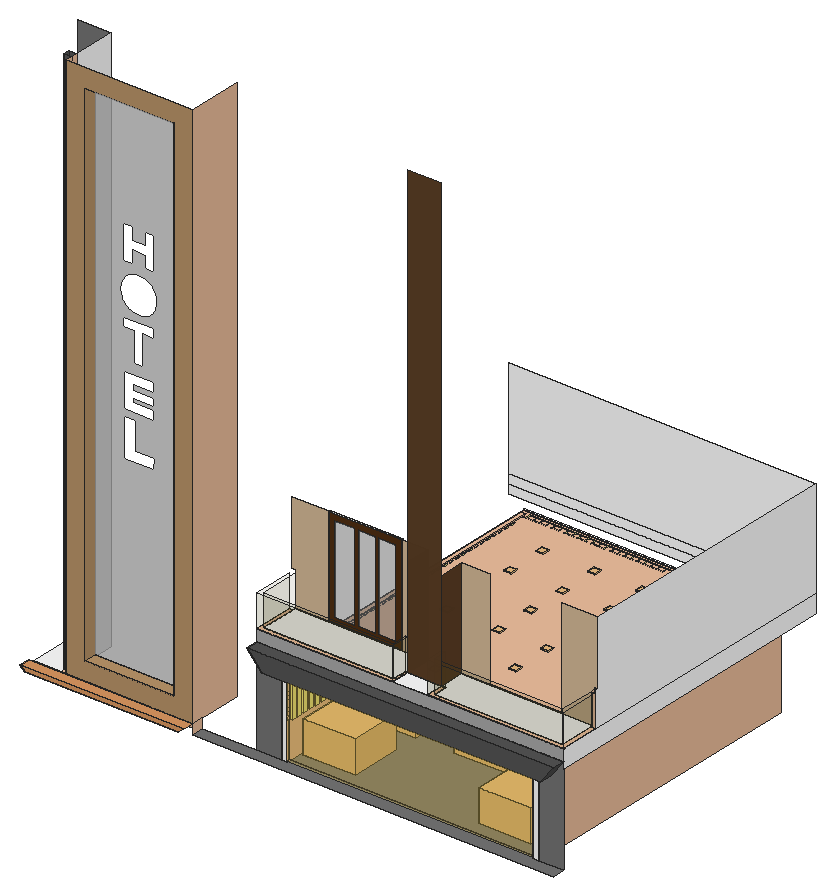
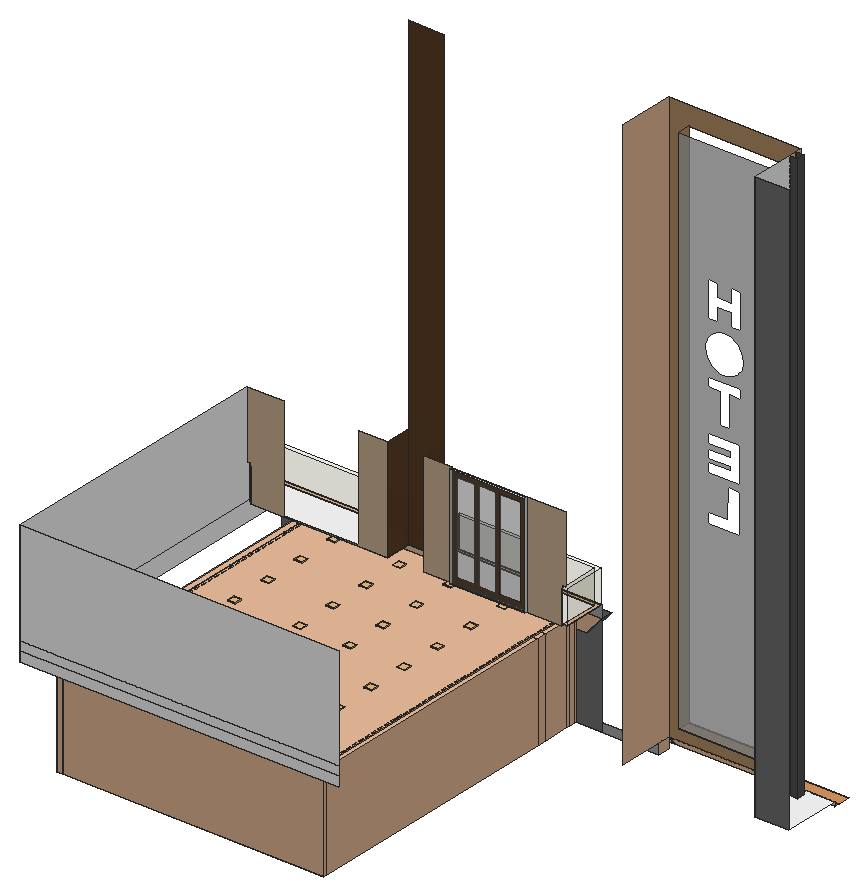
# SketchUp Ruby script. Lengths in inches.
U = 1.inch
M = Sketchup.active_model
def pt(a) = Geom::Point3d.new(a.map { |v| v * U })
def face(e, loops, mat)
  f = e.add_face(loops[0].map { |a| pt(a) })
  loops[1..].each { |l| e.add_face(l.map { |a| pt(a) }).erase! }
  f.material = f.back_material = mat if mat
  f
end
# faces: each face lists its corners as indices into pts; further lists are holes
def faces(e, pts, list, mat = nil) = list.each { |f| face(e, (f[0].is_a?(Array) ? f : [f]).map { |l| l.map { |i| pts[i] } }, mat) }
# xy, xz, yz: faces in a plane at the given z, y or x. An outline is a flat list of corners, or four numbers for a rectangle; further outlines are holes
def ring(l) = l.size == 4 ? [[l[0], l[1]], [l[2], l[1]], [l[2], l[3]], [l[0], l[3]]] : l.each_slice(2).to_a
def flat(e, list, mat, &to3) = list.each { |f| face(e, (f[0].is_a?(Array) ? f : [f]).map { |l| ring(l).map { |u, v| to3.(u, v) } }, mat) }
def xy(e, z, list, mat = nil) = flat(e, list, mat) { |x, y| [x, y, z] }
def xz(e, y, list, mat = nil) = flat(e, list, mat) { |x, z| [x, y, z] }
def yz(e, x, list, mat = nil) = flat(e, list, mat) { |y, z| [x, y, z] }
def lines(e, pts, list) = list.each { |a, b| e.add_line(pt(pts[a]), pt(pts[b])) }
# prism: a flat outline (further loops are holes) pulled along v
def prism(e, loops, v, mat = nil)
  f = face(e, loops, mat); d = Geom::Vector3d.new(v.map { |x| x * U })
  f.pushpull(f.normal.samedirection?(d) ? d.length : -d.length)
end
def box(e, o, s, mat = nil) = prism(e, [[o, [o[0] + s[0], o[1], o[2]], [o[0] + s[0], o[1] + s[1], o[2]], [o[0], o[1] + s[1], o[2]]]], [0, 0, s[2]], mat)
def at(x, y, z, deg = 0) = Geom::Transformation.translation(pt([x, y, z])) * Geom::Transformation.rotation(ORIGIN, Z_AXIS, deg.degrees)
def axes(o, x, y, z) = Geom::Transformation.new([*x, 0, *y, 0, *z, 0, *pt(o).to_a, 1])
def part(name) = M.definitions.add(name)
# library, detail: a bought-in or finely detailed component or shape, given as its bounding box
def library(name, o, s) = part(name).tap { |d| box(d.entities, o, s) }
def detail(e, o, s) = box(e.add_group.entities, o, s)
def put(e, d, t, mat = nil) = e.add_instance(d, t).tap { |i| i.material = mat if mat }
def group(e, t, mat = nil) = e.add_group.tap { |g| g.transformation = t; g.material = mat if mat }.entities
root = M.entities
M.materials.add("Generic\#1").color = [84, 84, 84]
M.materials.add("Generic\#10").color = [214, 187, 153]
M.materials.add("Generic\#12").color = [244, 243, 143]
M.materials.add("Generic\#13").color = [239, 192, 158]
M.materials.add("Generic\#14").color = [219, 152, 97]
M.materials.add("Generic\#3").color = [117, 117, 117]
M.materials.add("Generic\#4").color = [186, 149, 106]
M.materials.add("[Color M00]").color = [255, 255, 255]
M.materials.add("[Color M03]").color = [170, 170, 170]
M.materials.add("[Translucent Glass Dark Green]").color = [86, 83, 28]
M.materials["[Translucent Glass Dark Green]"].alpha = 0.11
M.materials.add("[Translucent Glass Gray]").color = [252, 208, 57]
M.materials["[Translucent Glass Gray]"].alpha = 0.16
M.materials.add("[Translucent Glass Gray]1").color = [127, 127, 127]
M.materials["[Translucent Glass Gray]1"].alpha = 0.3
M.materials.add("[Translucent Resin Crush Gray]").color = [183, 183, 183]
M.materials["[Translucent Resin Crush Gray]"].alpha = 0.8
M.materials.add("[Wood Bamboo]").color = [81, 48, 19]
M.materials.add("[Wood Floor]").color = [91, 62, 36]
M.materials["[Wood Floor]"].alpha = 0.99
c1 = library("cafe+table",[12.29,13.08,0],[75.61,73.69,46.46])
c2 = part("Group\#2")
xy(c2.entities,0,[[0,0,6,7.5]])
xz(c2.entities,0,[[0,0,6,78.75]])
yz(c2.entities,6,[[0,0,7.5,78.75]])
c3 = part("Group\#3")
xy(c3.entities,0,[[0,0,3.3125,5.875]])
xz(c3.entities,0,[[0,0,3.3125,78.75]])
xz(c3.entities,5.875,[[0,0,3.3125,78.75]])
yz(c3.entities,3.3125,[[0,0,5.875,78.75]])
c4 = part("Group\#4")
xy(c4.entities,0,[[0,0,3.6875,6.5625]])
xz(c4.entities,0,[[0,0,3.6875,78.75]])
yz(c4.entities,0,[[0,0,6.5625,78.75]])
c5 = library("Tlon Light 450 Ceiling 152 006",[-8.86,-8.86,-3.78],[17.72,17.72,3.56])
c6 = part("Group\#13")
xy(c6.entities,0,[[0,0,104.75,3]])
xy(c6.entities,142.8125,[[0,0,104.75,3]])
xz(c6.entities,0,[[8.08,8.08,37.11,134.73],[42.61,8.08,67.14,134.73],[72.39,8.08,96.67,134.73]],"[Translucent Glass Gray]1")
xz(c6.entities,0,[[[0,0,104.75,142.8125],[8.08,8.08,37.11,134.73],[42.61,8.08,67.14,134.73],[72.39,8.08,96.67,134.73]]],"[Wood Bamboo]")
xz(c6.entities,3,[[0,0,104.75,142.8125]],"[Translucent Glass Gray]1")
yz(c6.entities,0,[[0,0,3,142.8125]])
yz(c6.entities,104.75,[[0,0,3,142.8125]])
xy(root,168.25,[[440,78.3125,447.375,79.25],[803.1875,78.3125,812,515.9375],[440,79.25,447.375,88.375],[440,88.375,447.375,95.25],[440,95.25,447.375,130.75],
  [440,130.75,447.375,144.75],[440,144.75,447.375,510.9375],[440,510.9375,803.1875,515.9375]],"Generic\#13")
xy(root,168.25,[[324.25,60.4375,848,60.4375,848,78.3125,803.1875,78.3125,803.1875,510.9375,447.375,510.9375,447.375,78.3125,324.25,78.3125]],"Generic\#3")
xy(root,176.75,[[94.75,44.3125,316.0625,60.4375]],"Generic\#14")
xy(root,182.75,[[133.5625,60.4375,141.125,70.1875],[129.6875,70.1875,141.125,79.9375]],"Generic\#13")
xy(root,182.75,[[87.6875,44.3125,324.25,60.4375]],"Generic\#14")
xy(root,182.75,[[94.0625,60.4375,133.5625,60.4375,133.5625,70.1875,129.6875,70.1875,129.6875,79.9375,141.125,79.9375,141.125,140.75,94.0625,140.75]],"[Color M00]")
xy(root,209.65,[[168.02,60.4375,297.35,78.3125]],"Generic\#4")
xy(root,284,[[425.15,60.0625,829.58,78.3125]],"Generic\#1")
xy(root,300.625,[[440,78.3125,447.375,79.25],[447.375,78.3125,447.375,479.8125,450.6875,479.8125,450.6875,485.6875,447.375,485.6875,447.375,503.4375,453.375,503.4375,453.375,510.9375,803.1875,510.9375,803.1875,501.17,799.5,501.17,799.5,494.61,803.1875,494.61,803.1875,78.3125],[803.1875,78.3125,803.1875,494.61,799.5,494.61,799.5,501.17,803.1875,501.17,803.1875,515.9375,812,515.9375,812,78.3125],[440,79.25,447.375,88.375],[440,88.375,447.375,95.25],
  [440,95.25,447.375,130.75],[440,130.75,447.375,144.75],[440,144.75,447.375,510.9375],[447.375,479.8125,450.6875,485.6875],[447.375,503.4375,447.375,510.9375,440,510.9375,440,515.9375,803.1875,515.9375,803.1875,510.9375,453.375,510.9375,453.375,503.4375]],"Generic\#13")
xy(root,309.1875,[[404,60.0625,848,78.3125]],"Generic\#1")
xy(root,326.375,[[404,78.3125,404,136.9375,409.82,136.9375,409.82,83.375,598,83.375,598,104.5,601.0625,104.5,601.0625,78.3125],[650.9375,78.3125,650.9375,104.5,656.9375,104.5,656.9375,84.3125,842.4375,84.3125,842.4375,136.9375,848,136.9375,848,78.3125],[848,78.3125,848.4375,136.9375]],"Generic\#13")
xy(root,326.375,[[601.0625,78.3125,650.9375,104.5],[409.82,83.375,598,83.375,598,104.5,601.0625,104.5,601.0625,140.75,409.82,140.75],[656.9375,84.3125,842.4375,84.3125,842.4375,140.75,650.9375,140.75,650.9375,104.5,656.9375,104.5]],"[Color M00]")
xz(root,44.3125,[[94.75,176.75,316.0625,176.75,324.25,182.75,87.6875,182.75]],"Generic\#14")
xz(root,60.0625,[[425.15,284,829.58,284,848,309.1875,404,309.1875]],"Generic\#1")
xz(root,60.4375,[[94.0625,176.75,94.75,176.75,94.0625,177.34],[94.75,176.75,94.0625,177.34,94.0625,182.75,324.25,182.75,316.0625,176.75],[316.0625,176.75,324.25,176.75,324.25,182.75],[94.0625,177.34,87.6875,182.75,94.0625,182.75]],"Generic\#13")
xz(root,60.4375,[[[141.125,182.75,324.25,979.625],[168.02,209.65,297.35,952.73]]],"Generic\#4")
xz(root,70.1875,[[129.6875,182.75,141.125,979.625]],"Generic\#1")
xz(root,78.3125,[[425.15,284,404,309.1875,848,309.1875,829.58,284,812,284,812,300.625,440,300.625,440,284],[440,284,447.375,300.625],[447.375,284,803.1875,300.625],[803.1875,284,812,300.625]],"Generic\#13")
xz(root,78.3125,[[404,168.25,440,168.25,440,284,425.15,284,404,309.1875],[812,168.25,848,168.25,848,309.1875,829.58,284,812,284]],"Generic\#3")
xz(root,78.3125,[[440,168.25,447.375,284],[803.1875,168.25,812,284]],"[Color M00]")
xz(root,78.3125,[[404,309.1875,848,326.375]],"[Color M03]")
xz(root,78.3125,[[404,326.375,601.0625,372.75],[650.9375,326.375,848.4375,372.75]],"[Translucent Glass Dark Green]")
xz(root,78.3125,[[[168.02,209.65,297.35,952.73],[233.53,671.96,230.61,672.04,227.72,672.4375,224.88,673.16,222.15,674.19,219.55,675.53,217.11,677.14,214.875,679.02,212.86,681.14,211.1,683.47,209.61,685.98,208.4,688.65,207.51,691.43,206.93,694.3,206.68,697.21,206.75,700.13,207.15,703.02,207.875,705.86,208.91,708.59,210.24,711.19,211.86,713.625,213.74,715.86,215.86,717.88,218.1875,719.64,220.7,721.13,223.36,722.33,226.15,723.23,229.01,723.81,231.92,724.0625,234.84,723.99,237.74,723.59,240.57,722.87,243.3,721.83,245.91,720.5,248.34,718.88,250.58,717,252.59,714.88,254.36,712.55,255.85,710.04,257.05,707.375,257.95,704.59,258.52,701.73,258.78,698.82,258.7,695.9,258.3,693,257.58,690.17,256.55,687.44,255.21,684.83,253.6,682.4,251.72,680.16,249.6,678.15,247.27,676.38,244.76,674.89,242.09,673.69,239.27,672.93,236.44,672.22],[212.13,543.68,212.13,592.36,254.57,592.36,254.57,579.92,224.88,579.92,224.88,572.3,254.57,572.3,254.57,561.8,224.88,561.8,224.88,556.18,254.57,556.18,254.57,543.68],[210.88,735.92,210.88,783.92,222.88,783.92,222.88,765.92,242.57,765.92,242.57,783.92,254.57,783.92,254.57,735.92,242.57,735.92,242.57,753.92,222.88,753.92,222.88,735.92],[212.59,479.87,212.59,531.7,212.45,534.23,227.88,534.23,228.04,494.05,254.73,494.05,254.57,479.87],[226.26,608.06,226.26,650.42,210.88,650.42,210.88,662.42,254.57,662.42,254.57,650.42,238.26,650.42,238.26,608.06]]],"[Translucent Resin Crush Gray]")
xz(root,79.25,[[440,168.25,447.375,300.625]],"Generic\#13")
xz(root,79.9375,[[129.6875,182.75,141.125,979.625]],"Generic\#1")
xz(root,83.375,[[409.82,326.375,598,372.75]],"[Translucent Glass Dark Green]")
xz(root,84.3125,[[656.9375,326.375,842.4375,372.75]],"[Translucent Glass Dark Green]")
xz(root,104.5,[[598,326.375,601.0625,372.75],[650.9375,326.375,656.9375,372.75]],"[Translucent Glass Dark Green]")
xz(root,104.5,[[601.0625,326.375,650.9375,979.625]],"[Wood Floor]")
xz(root,136.9375,[[842.4375,326.375,848,372.75]],"Generic\#13")
xz(root,136.9375,[[848,326.375,848.4375,372.75]],"[Translucent Glass Dark Green]")
xz(root,140.75,[[409.82,326.375,601.0625,326.375,601.0625,470.375,562.95,470.375,562.95,327.5625,458.2,327.5625,458.2,470.375,404,470.375,404,377.0625,409.82,377.0625],[650.9375,326.375,842.4375,326.375,842.4375,377.0625,848,377.0625,848,470.375,795.95,470.375,795.95,327.5625,691.2,327.5625,691.2,470.375,650.9375,470.375]],"Generic\#10")
xz(root,140.75,[[94.0625,182.75,141.125,979.625]],"Generic\#3")
xz(root,501.17,[[799.5,221.875,803.1875,300.625]],"Generic\#13")
xz(root,510.9375,[[440,168.25,447.375,300.625],[447.375,168.25,803.1875,221.875],[453.375,221.875,803.1875,300.625]],"Generic\#13")
xz(root,515.9375,[[440,168.25,803.1875,300.625],[803.1875,168.25,812,300.625]],"Generic\#13")
xz(root,534.3125,[[404,300.625,848,313.75],[404,313.75,848,326.375],[404,326.375,848,470.375]],"[Color M00]")
yz(root,129.6875,[[70.1875,182.75,79.9375,979.625]],"Generic\#1")
yz(root,141.125,[[60.4375,182.75,70.1875,979.625],[70.1875,182.75,79.9375,979.625]],"Generic\#13")
yz(root,141.125,[[79.9375,182.75,140.75,979.625]],"[Color M00]")
yz(root,168.02,[[60.4375,209.65,78.3125,952.73]],"Generic\#4")
yz(root,297.35,[[60.4375,209.65,78.3125,952.73]],"Generic\#4")
yz(root,324.25,[[60.4375,168.25,78.3125,182.75],[60.4375,182.75,140.75,979.625]],"Generic\#13")
yz(root,404,[[78.3125,326.375,136.9375,372.75]],"[Translucent Glass Dark Green]")
yz(root,409.82,[[83.375,326.375,140.75,372.75]],"[Translucent Glass Dark Green]")
yz(root,440,[[78.3125,168.25,79.25,300.625],[79.25,168.25,88.375,300.625],[88.375,168.25,95.25,300.625],[95.25,168.25,130.75,300.625],[130.75,168.25,144.75,300.625],
  [144.75,168.25,510.9375,300.625],[510.9375,168.25,515.9375,300.625]],"Generic\#13")
yz(root,447.375,[[78.3125,168.25,79.25,221.875],[79.25,168.25,510.9375,221.875],[78.3125,221.875,79.25,284],[79.25,221.875,88.375,300.625],[88.375,221.875,95.25,300.625],
  [95.25,221.875,130.75,300.625],[130.75,221.875,144.75,300.625],[144.75,221.875,479.8125,300.625],[479.8125,221.875,485.6875,300.625],[485.6875,221.875,503.4375,300.625],
  [503.4375,221.875,510.9375,300.625],[78.3125,284,79.25,300.625]],"Generic\#13")
yz(root,598,[[83.375,326.375,104.5,372.75]],"[Translucent Glass Dark Green]")
yz(root,601.0625,[[78.3125,326.375,104.5,372.75]],"[Translucent Glass Dark Green]")
yz(root,601.0625,[[104.5,326.375,140.75,470.375]],"[Wood Floor]")
yz(root,650.9375,[[78.3125,326.375,104.5,372.75]],"[Translucent Glass Dark Green]")
yz(root,650.9375,[[104.5,326.375,140.75,470.375]],"[Wood Floor]")
yz(root,656.9375,[[84.3125,326.375,104.5,372.75]],"[Translucent Glass Dark Green]")
yz(root,803.1875,[[78.3125,168.25,510.9375,221.875],[510.9375,168.25,515.9375,300.625],[78.3125,221.875,494.61,300.625],[501.17,221.875,510.9375,300.625]],"Generic\#13")
yz(root,812,[[78.3125,168.25,515.9375,300.625]],"Generic\#13")
yz(root,842.4375,[[136.9375,326.375,140.75,372.75]],"Generic\#13")
yz(root,842.4375,[[84.3125,326.375,136.9375,372.75]],"[Translucent Glass Dark Green]")
yz(root,848,[[78.3125,300.625,534.3125,326.375],[136.9375,326.375,534.3125,326.375,534.3125,470.375,140.75,470.375,140.75,377.0625,136.9375,377.0625]],"[Color M00]")
yz(root,848.4375,[[78.3125,326.375,136.9375,372.75]],"[Translucent Glass Dark Green]")
p = [[94.75,44.3125,176.75],[87.6875,44.3125,182.75],[87.6875,60.4375,182.75],[94.0625,60.4375,177.34],[94.75,60.4375,176.75],[324.25,44.3125,182.75],
  [316.0625,44.3125,176.75],[316.0625,60.4375,176.75],[324.25,60.4375,182.75],[425.15,60.0625,284],[404,60.0625,309.1875],[404,78.3125,309.1875],
  [425.15,78.3125,284],[848,60.0625,309.1875],[829.58,60.0625,284],[829.58,78.3125,284],[848,78.3125,309.1875],[440,515.9375,303.1875],
  [812,515.9375,303.1875],[447.375,73.3125,300.625],[447.375,78.3125,300.625]]
faces(root,p,[[0,1,2,3,4],[5,6,7,8]],"Generic\#14")
faces(root,p,[[9,10,11,12],[13,14,15,16]],"Generic\#1")
lines(root,p,[[17,18],[19,20]])
g1 = group(root,at(447.375,78.3125,168.25))
box(g1,[0,0,0],[355.8125,5,115.75],"[Translucent Glass Gray]")
put(root,c1,at(696.0625,404.72,171.375))
put(root,c1,at(442,404.72,171.375))
put(root,c1,at(442,195.28,171.375))
put(root,c1,at(696.0625,195.28,171.375))
put(root,c1,at(573.0625,195.28,171.375))
put(root,c1,at(442,292.03,171.375))
put(root,c1,at(573.0625,292.03,171.375))
put(root,c1,at(696.0625,292.03,171.375))
put(root,c1,at(573.0625,404.72,171.375))
put(root,c1,at(442,85.59,171.375))
put(root,c1,at(696.0625,85.59,171.375))
put(root,c2,at(447.375,503.4375,221.875),"Generic\#12")
put(root,c2,at(456.8125,503.4375,221.875),"Generic\#12")
put(root,c2,at(466.25,503.4375,221.875),"Generic\#12")
put(root,c2,at(475.6875,503.4375,221.875),"Generic\#12")
put(root,c2,at(485.125,503.4375,221.875),"Generic\#12")
put(root,c2,at(494.5625,503.4375,221.875),"Generic\#12")
put(root,c2,at(504,503.4375,221.875),"Generic\#12")
put(root,c2,at(513.4375,503.4375,221.875),"Generic\#12")
put(root,c2,at(522.875,503.4375,221.875),"Generic\#12")
put(root,c2,at(532.3125,503.4375,221.875),"Generic\#12")
put(root,c2,at(541.75,503.4375,221.875),"Generic\#12")
put(root,c2,at(551.1875,503.4375,221.875),"Generic\#12")
put(root,c2,at(560.625,503.4375,221.875),"Generic\#12")
put(root,c2,at(570.0625,503.4375,221.875),"Generic\#12")
put(root,c2,at(579.5,503.4375,221.875),"Generic\#12")
put(root,c2,at(588.9375,503.4375,221.875),"Generic\#12")
put(root,c2,at(598.375,503.4375,221.875),"Generic\#12")
put(root,c2,at(607.8125,503.4375,221.875),"Generic\#12")
put(root,c2,at(617.25,503.4375,221.875),"Generic\#12")
put(root,c2,at(626.6875,503.4375,221.875),"Generic\#12")
put(root,c2,at(636.125,503.4375,221.875),"Generic\#12")
put(root,c2,at(645.5625,503.4375,221.875),"Generic\#12")
put(root,c2,at(655,503.4375,221.875),"Generic\#12")
put(root,c2,at(664.4375,503.4375,221.875),"Generic\#12")
put(root,c2,at(673.875,503.4375,221.875),"Generic\#12")
put(root,c2,at(683.3125,503.4375,221.875),"Generic\#12")
put(root,c2,at(692.75,503.4375,221.875),"Generic\#12")
put(root,c2,at(702.1875,503.4375,221.875),"Generic\#12")
put(root,c2,at(711.625,503.4375,221.875),"Generic\#12")
put(root,c2,at(721.0625,503.4375,221.875),"Generic\#12")
put(root,c2,at(730.5,503.4375,221.875),"Generic\#12")
put(root,c2,at(739.9375,503.4375,221.875),"Generic\#12")
put(root,c2,at(749.375,503.4375,221.875),"Generic\#12")
put(root,c2,at(758.8125,503.4375,221.875),"Generic\#12")
put(root,c2,at(768.25,503.4375,221.875),"Generic\#12")
put(root,c2,at(777.6875,503.4375,221.875),"Generic\#12")
put(root,c2,at(786.01,503.4375,221.875),"Generic\#12")
put(root,c2,at(794.34,503.4375,221.875),"Generic\#12")
put(root,c3,at(447.375,479.8125,221.875),"Generic\#12")
put(root,c3,at(447.375,468.75,221.875),"Generic\#12")
put(root,c3,at(447.375,457.6875,221.875),"Generic\#12")
put(root,c3,at(447.375,446.625,221.875),"Generic\#12")
put(root,c3,at(447.375,435.5625,221.875),"Generic\#12")
put(root,c3,at(447.375,424.5,221.875),"Generic\#12")
put(root,c3,at(447.375,413.4375,221.875),"Generic\#12")
put(root,c3,at(447.375,402.375,221.875),"Generic\#12")
put(root,c3,at(447.375,391.3125,221.875),"Generic\#12")
put(root,c3,at(447.375,380.25,221.875),"Generic\#12")
put(root,c3,at(447.375,369.1875,221.875),"Generic\#12")
put(root,c3,at(447.375,358.125,221.875),"Generic\#12")
put(root,c3,at(447.375,347.0625,221.875),"Generic\#12")
put(root,c3,at(447.375,336,221.875),"Generic\#12")
put(root,c3,at(447.375,324.9375,221.875),"Generic\#12")
put(root,c3,at(447.375,313.875,221.875),"Generic\#12")
put(root,c3,at(447.375,302.8125,221.875),"Generic\#12")
put(root,c3,at(447.375,291.75,221.875),"Generic\#12")
put(root,c3,at(447.375,280.6875,221.875),"Generic\#12")
put(root,c3,at(447.375,269.625,221.875),"Generic\#12")
put(root,c3,at(447.375,258.5625,221.875),"Generic\#12")
put(root,c3,at(447.375,247.5,221.875),"Generic\#12")
put(root,c3,at(447.375,236.4375,221.875),"Generic\#12")
put(root,c3,at(447.375,225.375,221.875),"Generic\#12")
put(root,c3,at(447.375,214.3125,221.875),"Generic\#12")
put(root,c3,at(447.375,203.25,221.875),"Generic\#12")
put(root,c3,at(447.375,192.1875,221.875),"Generic\#12")
put(root,c3,at(447.375,181.125,221.875),"Generic\#12")
put(root,c3,at(447.375,170.0625,221.875),"Generic\#12")
put(root,c3,at(447.375,159,221.875),"Generic\#12")
put(root,c3,at(447.375,147.9375,221.875),"Generic\#12")
put(root,c3,at(447.375,136.875,221.875),"Generic\#12")
put(root,c3,at(447.375,125.8125,221.875),"Generic\#12")
put(root,c3,at(447.375,114.75,221.875),"Generic\#12")
put(root,c3,at(447.375,103.6875,221.875),"Generic\#12")
put(root,c3,at(447.375,92.625,221.875),"Generic\#12")
put(root,c3,at(447.375,83.4375,221.875),"Generic\#12")
put(root,c4,at(799.5,494.61,221.875),"Generic\#12")
put(root,c4,at(799.5,482.91,221.875),"Generic\#12")
put(root,c4,at(799.5,471.21,221.875),"Generic\#12")
put(root,c4,at(799.5,459.51,221.875),"Generic\#12")
put(root,c4,at(799.5,447.81,221.875),"Generic\#12")
put(root,c4,at(799.5,436.11,221.875),"Generic\#12")
put(root,c4,at(799.5,424.41,221.875),"Generic\#12")
put(root,c4,at(799.5,412.7,221.875),"Generic\#12")
put(root,c4,at(799.5,401,221.875),"Generic\#12")
put(root,c4,at(799.5,389.3,221.875),"Generic\#12")
put(root,c4,at(799.5,377.6,221.875),"Generic\#12")
put(root,c4,at(799.5,365.9,221.875),"Generic\#12")
put(root,c4,at(799.5,354.2,221.875),"Generic\#12")
put(root,c4,at(799.5,342.5,221.875),"Generic\#12")
put(root,c4,at(799.5,330.8,221.875),"Generic\#12")
put(root,c4,at(799.5,319.1,221.875),"Generic\#12")
put(root,c4,at(799.5,307.4,221.875),"Generic\#12")
put(root,c4,at(799.5,295.7,221.875),"Generic\#12")
put(root,c4,at(799.5,284,221.875),"Generic\#12")
put(root,c4,at(799.5,272.3,221.875),"Generic\#12")
put(root,c4,at(799.5,260.6,221.875),"Generic\#12")
put(root,c4,at(799.5,248.9,221.875),"Generic\#12")
put(root,c4,at(799.5,237.19,221.875),"Generic\#12")
put(root,c4,at(799.5,225.49,221.875),"Generic\#12")
put(root,c4,at(799.5,213.79,221.875),"Generic\#12")
put(root,c4,at(799.5,202.09,221.875),"Generic\#12")
put(root,c4,at(799.5,190.39,221.875),"Generic\#12")
put(root,c4,at(799.5,178.69,221.875),"Generic\#12")
put(root,c4,at(799.5,166.99,221.875),"Generic\#12")
put(root,c4,at(799.5,155.29,221.875),"Generic\#12")
put(root,c4,at(799.5,143.59,221.875),"Generic\#12")
put(root,c4,at(799.5,131.89,221.875),"Generic\#12")
put(root,c4,at(799.5,120.1875,221.875),"Generic\#12")
put(root,c4,at(799.5,108.49,221.875),"Generic\#12")
put(root,c4,at(799.5,96.79,221.875),"Generic\#12")
put(root,c4,at(799.5,85.09,221.875),"Generic\#12")
put(root,c5,axes([751.05,109.4375,301.44],[0.6,0,0],[0,0.6,0],[0,0,0.6]))
put(root,c5,axes([751.05,167.1875,301.44],[0.6,0,0],[0,0.6,0],[0,0,0.6]))
put(root,c5,axes([751.05,224.9375,301.44],[0.6,0,0],[0,0.6,0],[0,0,0.6]))
put(root,c5,axes([751.05,282.6875,301.44],[0.6,0,0],[0,0.6,0],[0,0,0.6]))
put(root,c5,axes([751.05,340.4375,301.44],[0.6,0,0],[0,0.6,0],[0,0,0.6]))
put(root,c5,axes([751.05,398.1875,301.44],[0.6,0,0],[0,0.6,0],[0,0,0.6]))
put(root,c5,axes([751.05,455.9375,301.44],[0.6,0,0],[0,0.6,0],[0,0,0.6]))
put(root,c5,axes([660.36,109.4375,301.44],[0.6,0,0],[0,0.6,0],[0,0,0.6]))
put(root,c5,axes([660.36,167.1875,301.44],[0.6,0,0],[0,0.6,0],[0,0,0.6]))
put(root,c5,axes([660.36,398.1875,301.44],[0.6,0,0],[0,0.6,0],[0,0,0.6]))
put(root,c5,axes([660.36,282.6875,301.44],[0.6,0,0],[0,0.6,0],[0,0,0.6]))
put(root,c5,axes([660.36,224.9375,301.44],[0.6,0,0],[0,0.6,0],[0,0,0.6]))
put(root,c5,axes([660.36,455.9375,301.44],[0.6,0,0],[0,0.6,0],[0,0,0.6]))
put(root,c5,axes([660.36,340.4375,301.44],[0.6,0,0],[0,0.6,0],[0,0,0.6]))
put(root,c5,axes([590.55,398.1875,301.44],[0.6,0,0],[0,0.6,0],[0,0,0.6]))
put(root,c5,axes([590.55,282.6875,301.44],[0.6,0,0],[0,0.6,0],[0,0,0.6]))
put(root,c5,axes([590.55,109.4375,301.44],[0.6,0,0],[0,0.6,0],[0,0,0.6]))
put(root,c5,axes([590.55,167.1875,301.44],[0.6,0,0],[0,0.6,0],[0,0,0.6]))
put(root,c5,axes([590.55,224.9375,301.44],[0.6,0,0],[0,0.6,0],[0,0,0.6]))
put(root,c5,axes([590.55,455.9375,301.44],[0.6,0,0],[0,0.6,0],[0,0,0.6]))
put(root,c5,axes([590.55,340.4375,301.44],[0.6,0,0],[0,0.6,0],[0,0,0.6]))
put(root,c5,axes([515.17,398.1875,301.44],[0.6,0,0],[0,0.6,0],[0,0,0.6]))
put(root,c5,axes([515.17,455.9375,301.44],[0.6,0,0],[0,0.6,0],[0,0,0.6]))
put(root,c5,axes([515.17,167.1875,301.44],[0.6,0,0],[0,0.6,0],[0,0,0.6]))
put(root,c5,axes([515.17,340.4375,301.44],[0.6,0,0],[0,0.6,0],[0,0,0.6]))
put(root,c5,axes([515.17,224.9375,301.44],[0.6,0,0],[0,0.6,0],[0,0,0.6]))
put(root,c5,axes([515.17,109.4375,301.44],[0.6,0,0],[0,0.6,0],[0,0,0.6]))
put(root,c5,axes([515.17,282.6875,301.44],[0.6,0,0],[0,0.6,0],[0,0,0.6]))
put(root,c6,at(458.2,140.75,326.375))
